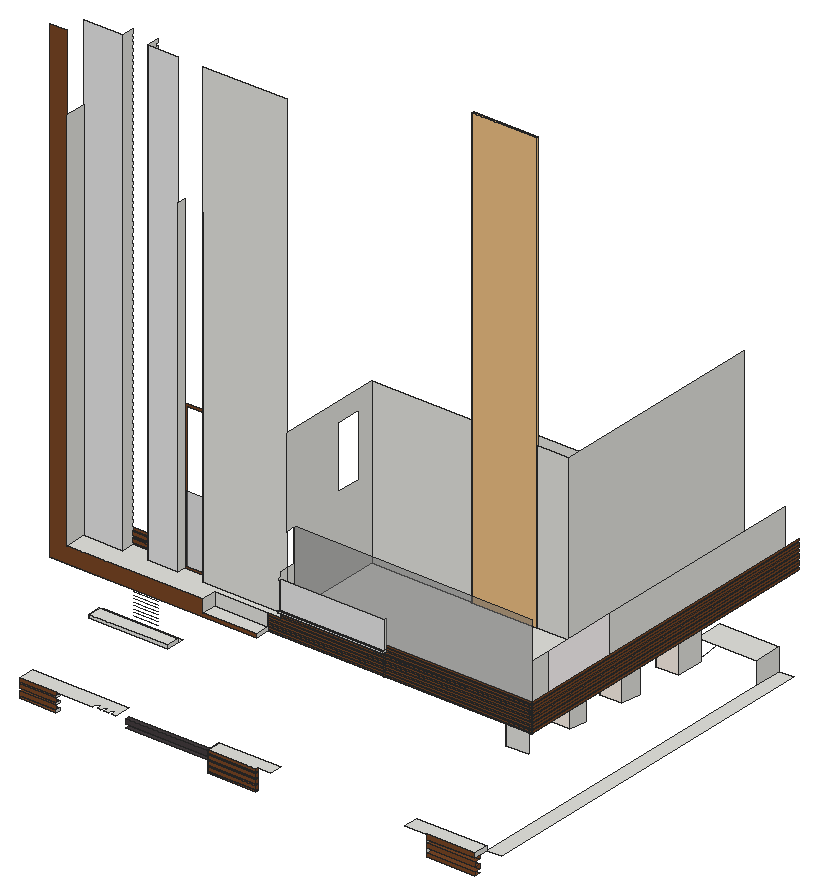
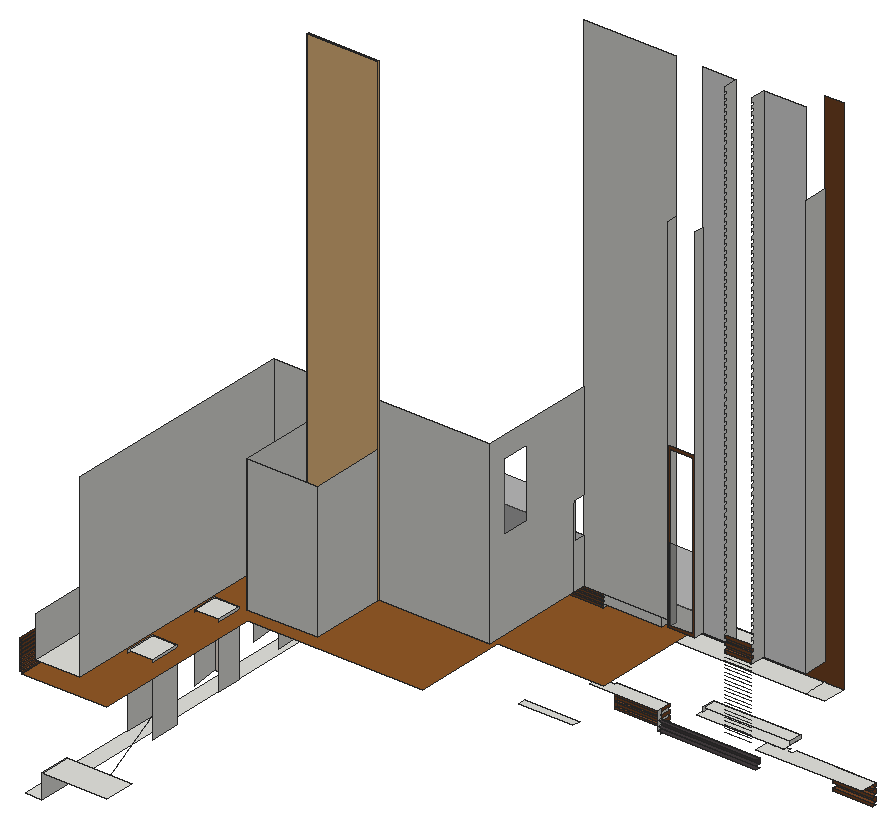
# SketchUp Ruby script. Lengths in inches.
U = 1.inch
M = Sketchup.active_model
def pt(a) = Geom::Point3d.new(a.map { |v| v * U })
def face(e, loops, mat)
  f = e.add_face(loops[0].map { |a| pt(a) })
  loops[1..].each { |l| e.add_face(l.map { |a| pt(a) }).erase! }
  f.material = f.back_material = mat if mat
  f
end
# faces: each face lists its corners as indices into pts; further lists are holes
def faces(e, pts, list, mat = nil) = list.each { |f| face(e, (f[0].is_a?(Array) ? f : [f]).map { |l| l.map { |i| pts[i] } }, mat) }
# xy, xz, yz: faces in a plane at the given z, y or x. An outline is a flat list of corners, or four numbers for a rectangle; further outlines are holes
def ring(l) = l.size == 4 ? [[l[0], l[1]], [l[2], l[1]], [l[2], l[3]], [l[0], l[3]]] : l.each_slice(2).to_a
def flat(e, list, mat, &to3) = list.each { |f| face(e, (f[0].is_a?(Array) ? f : [f]).map { |l| ring(l).map { |u, v| to3.(u, v) } }, mat) }
def xy(e, z, list, mat = nil) = flat(e, list, mat) { |x, y| [x, y, z] }
def xz(e, y, list, mat = nil) = flat(e, list, mat) { |x, z| [x, y, z] }
def yz(e, x, list, mat = nil) = flat(e, list, mat) { |y, z| [x, y, z] }
def lines(e, pts, list) = list.each { |a, b| e.add_line(pt(pts[a]), pt(pts[b])) }
# prism: a flat outline (further loops are holes) pulled along v
def prism(e, loops, v, mat = nil)
  f = face(e, loops, mat); d = Geom::Vector3d.new(v.map { |x| x * U })
  f.pushpull(f.normal.samedirection?(d) ? d.length : -d.length)
end
def box(e, o, s, mat = nil) = prism(e, [[o, [o[0] + s[0], o[1], o[2]], [o[0] + s[0], o[1] + s[1], o[2]], [o[0], o[1] + s[1], o[2]]]], [0, 0, s[2]], mat)
def at(x, y, z, deg = 0) = Geom::Transformation.translation(pt([x, y, z])) * Geom::Transformation.rotation(ORIGIN, Z_AXIS, deg.degrees)
def axes(o, x, y, z) = Geom::Transformation.new([*x, 0, *y, 0, *z, 0, *pt(o).to_a, 1])
def part(name) = M.definitions.add(name)
# library, detail: a bought-in or finely detailed component or shape, given as its bounding box
def library(name, o, s) = part(name).tap { |d| box(d.entities, o, s) }
def detail(e, o, s) = box(e.add_group.entities, o, s)
def put(e, d, t, mat = nil) = e.add_instance(d, t).tap { |i| i.material = mat if mat }
def group(e, t, mat = nil) = e.add_group.tap { |g| g.transformation = t; g.material = mat if mat }.entities
root = M.entities
M.materials.add("[0009_Linen]").color = [250, 240, 230]
M.materials.add("[0010_Snow]").color = [255, 250, 250]
M.materials.add("[Asphalt New]").color = [67, 60, 62]
M.materials.add("[Polished Concrete Old]").color = [229, 229, 229]
M.materials.add("[Translucent Glass Gray]").color = [128, 128, 128]
M.materials["[Translucent Glass Gray]"].alpha = 0.5
M.materials.add("[Wood Floor Parquet]").color = [145, 89, 39]
M.materials.add("[Wood Veneer 01]").color = [120, 70, 37]
c1 = library("Stacked entry doors",[0,-1.38,0],[114.46,3.16,780.57])
xy(root,87.39,[[455.17,254.69,541.39,258.13]],"[Wood Veneer 01]")
xy(root,87.68,[[842.13,258.13,927.67,268.51]],"[Wood Veneer 01]")
xy(root,90.67,[[455.17,254.69,541.39,258.13]],"[Wood Veneer 01]")
xy(root,91.81,[[124.44,250.88,189.05,258.13]],"[Wood Veneer 01]")
xy(root,93.96,[[842.13,258.13,927.67,268.51]],"[Wood Veneer 01]")
xy(root,94.84,[[295.6,273.26,455.17,279.68]],"[Asphalt New]")
xy(root,96.21,[[124.44,250.88,189.05,258.13]],"[Wood Veneer 01]")
xy(root,97.01,[[455.17,254.69,541.39,258.13]],"[Wood Veneer 01]")
xy(root,99.55,[[455.17,254.69,541.39,258.13]],"[Wood Veneer 01]")
xy(root,100.52,[[295.6,273.26,455.17,279.68]],"[Asphalt New]")
xy(root,101.99,[[842.13,258.13,927.67,268.51]],"[Wood Veneer 01]")
xy(root,103.18,[[124.44,250.88,189.05,258.13]],"[Wood Veneer 01]")
xy(root,105.89,[[455.17,254.69,541.39,258.13]],"[Wood Veneer 01]")
xy(root,107.59,[[124.44,250.88,189.05,258.13]],"[Wood Veneer 01]")
xy(root,108.92,[[455.17,254.69,541.39,258.13]],"[Wood Veneer 01]")
xy(root,109.42,[[295.6,273.26,455.17,279.68]],"[Asphalt New]")
xy(root,109.73,[[842.13,258.13,927.67,268.51]],"[Wood Veneer 01]")
xy(root,114.56,[[124.44,250.88,189.05,258.13]],"[Wood Veneer 01]")
xy(root,115.26,[[455.17,254.69,541.39,258.13]],"[Wood Veneer 01]")
xy(root,116.625,[[927.67,284.25,954.26,934.03]])
xy(root,117.42,[[124.44,250.88,189.05,258.13]],"[Wood Veneer 01]")
xy(root,118.74,[[455.17,254.69,541.39,258.13]],"[Wood Veneer 01]")
xy(root,124,[[124.44,250.88,253.79,250.88,253.79,258.13,262.32,258.13,262.32,250.88,268.72,250.88,268.72,258.13,274.39,258.13,274.39,250.88,281.75,250.88,281.75,258.13,287.33,258.13,287.33,250.88,295.6,250.88,295.6,279.68,124.44,279.68],[455.17,254.69,541.39,254.69,541.39,258.13,565.2,258.13,565.2,279.68,455.17,279.68],[803.4375,258.13,927.67,284.25]])
xy(root,155.125,[[821.9,884.53,927.67,934.03]])
xy(root,203.35,[[181.21,332.61,321.33,367.17]])
xy(root,209.22,[[181.21,332.61,321.33,354.61]])
xy(root,222.18,[[406.18,498.96,495.01,511.34]])
xy(root,284.1875,[[850.45,424,889.83,460.43]])
xy(root,284.375,[[850.45,516.77,889.83,551.84]])
xy(root,287.75,[[124.44,316.98,154.8,354.61],[154.8,316.98,366.22,354.61]])
xy(root,287.75,[[366.22,316.98,492.15,316.98,492.15,342.73,960.69,342.73,960.69,934.03,821.9,934.03,821.9,649.35,538.78,649.35,538.78,498.96,366.22,498.96]],"[Wood Floor Parquet]")
xy(root,290.83,[[850.45,631.85,889.83,672.61],[850.45,757.51,889.83,807.18]])
xy(root,290.83,[[492.15,342.29,701.8,342.73],[701.8,342.29,960.69,342.73],[960.69,342.73,962.51,934.03]],"[Wood Veneer 01]")
xy(root,293.61,[[397.15,316.98,492.15,342.73]])
xy(root,294,[[701.8,342.29,960.69,342.73],[960.69,342.73,962.51,934.03]],"[Wood Veneer 01]")
xy(root,296.52,[[492.15,342.29,701.8,342.73],[701.8,342.29,960.69,342.73],[960.69,342.73,962.51,934.03]],"[Wood Veneer 01]")
xy(root,299.69,[[492.15,342.29,701.8,342.73],[701.8,342.29,960.69,342.73],[960.69,342.73,962.51,934.03]],"[Wood Veneer 01]")
xy(root,302.21,[[492.15,342.29,701.8,342.73],[701.8,342.29,960.69,342.73],[960.69,342.73,962.51,934.03]],"[Wood Veneer 01]")
xy(root,305.38,[[492.15,342.29,701.8,342.73],[701.8,342.29,960.69,342.73],[960.69,342.73,962.51,934.03]],"[Wood Veneer 01]")
xy(root,307.89,[[492.15,342.29,701.8,342.73],[701.8,342.29,960.69,342.73],[960.69,342.73,962.51,934.03]],"[Wood Veneer 01]")
xy(root,311.07,[[492.15,342.29,701.8,342.73],[701.8,342.29,960.69,342.73],[960.69,342.73,962.51,934.03]],"[Wood Veneer 01]")
xy(root,313.58,[[492.15,342.29,701.8,342.73],[701.8,342.29,960.69,342.73],[960.69,342.73,962.51,934.03]],"[Wood Veneer 01]")
xy(root,316.375,[[154.8,316.98,397.15,316.98,397.15,342.73,492.15,342.73,492.15,342.29,515.24,342.29,515.24,354.61,366.22,354.61,366.22,370.17,322.47,370.17,322.47,354.61,268.36,354.61,268.36,378.04,224.18,378.04,224.18,354.61,154.8,354.61],[515.24,373.53,937.99,373.53,937.99,543.54,810.09,543.54,810.09,667.11,695.625,667.11,695.625,543.54,515.24,543.54],[865.61,543.54,937.99,934.03]])
xy(root,316.75,[[701.8,342.29,960.69,342.73],[960.69,342.73,962.51,934.03]],"[Wood Veneer 01]")
xy(root,319.27,[[515.24,342.29,701.8,342.73],[701.8,342.29,960.69,342.73],[960.69,342.73,962.51,934.03]],"[Wood Veneer 01]")
xy(root,321.94,[[224.18,374.04,268.36,378.04]],"[Wood Veneer 01]")
xy(root,322.44,[[515.24,342.29,701.8,342.73],[701.8,342.29,960.69,342.73],[960.69,342.73,962.51,934.03]],"[Wood Veneer 01]")
xy(root,324.96,[[515.24,342.29,701.8,342.73],[701.8,342.29,960.69,342.73],[960.69,342.73,962.51,934.03]],"[Wood Veneer 01]")
xy(root,327.89,[[515.24,336.36,701.8,342.29]])
xy(root,327.96,[[224.18,374.04,268.36,378.04]],"[Wood Veneer 01]")
xy(root,328.13,[[701.8,342.29,960.69,342.73],[960.69,342.73,962.51,934.03]],"[Wood Veneer 01]")
xy(root,330.375,[[515.24,336.36,701.8,339.61]])
xy(root,330.64,[[701.8,342.29,960.69,342.73],[960.69,342.73,962.51,934.03]],"[Wood Veneer 01]")
xy(root,332.82,[[224.18,374.04,268.36,378.04]],"[Wood Veneer 01]")
xy(root,333.82,[[701.8,342.29,960.69,342.73],[960.69,342.73,962.51,934.03]],"[Wood Veneer 01]")
xy(root,336.33,[[701.8,342.29,960.69,342.73],[960.69,342.73,962.51,934.03]],"[Wood Veneer 01]")
xy(root,338.84,[[224.18,374.04,268.36,378.04]],"[Wood Veneer 01]")
xz(root,250.88,[[124.44,96.21,189.05,103.18],[124.44,107.59,189.05,114.56],[124.44,117.42,189.05,124]],"[Wood Veneer 01]")
xz(root,254.69,[[455.17,90.67,541.39,97.01],[455.17,99.55,541.39,105.89],[455.17,108.92,541.39,115.26],[455.17,118.74,541.39,124]],"[Wood Veneer 01]")
xz(root,258.13,[[455.17,87.39,541.39,90.67],[842.13,87.68,927.67,93.96],[124.44,91.81,189.05,96.21],[455.17,97.01,541.39,99.55],[842.13,101.99,927.67,109.73],
  [124.44,103.18,189.05,107.59],[455.17,105.89,541.39,108.92],[124.44,114.56,189.05,117.42],[455.17,115.26,541.39,118.74],[842.13,115.72,927.67,116.625,927.67,124,842.13,124]],"[Wood Veneer 01]")
xz(root,268.51,[[842.13,93.96,927.67,101.99],[842.13,109.73,927.67,109.73,927.67,116.625,842.13,115.72]],"[Wood Veneer 01]")
xz(root,273.26,[[295.6,100.52,455.17,109.42]],"[Asphalt New]")
xz(root,316.98,[[124.44,287.75,492.15,287.75,492.15,293.61,397.15,293.61,397.15,316.375,154.8,316.375,154.8,1137.19,124.44,1137.19]],"[Wood Veneer 01]")
xz(root,332.61,[[181.21,203.35,321.33,209.22]])
xz(root,336.36,[[515.24,327.89,701.8,330.375]],"[Polished Concrete Old]")
xz(root,339.61,[[515.24,330.375,701.8,380.42]],"[Polished Concrete Old]")
xz(root,342.29,[[492.15,290.83,701.8,290.83,701.8,294,492.15,293.61],[701.8,290.83,960.69,294],[492.15,296.52,701.8,299.69],[701.8,296.52,960.69,299.69],[492.15,302.21,701.8,305.38],
  [701.8,302.21,960.69,305.38],[492.15,307.89,701.8,311.07],[701.8,307.89,960.69,311.07],[492.15,313.58,701.8,313.58,701.8,316.75,515.24,316.375,492.15,316.375],[701.8,313.58,960.69,316.75],
  [515.24,319.27,701.8,322.44],[701.8,319.27,960.69,322.44],[515.24,324.96,701.8,327.89],[701.8,324.96,960.69,328.13],[701.8,330.64,960.69,333.82],
  [701.8,336.33,960.69,339.5]],"[Wood Veneer 01]")
xz(root,342.73,[[397.15,293.61,492.15,316.375]])
xz(root,342.73,[[492.15,287.75,701.8,288.32],[701.8,287.75,960.69,288.32],[492.15,288.32,701.8,290.83],[701.8,288.32,960.69,290.83],[960.69,290.83,962.51,294],
  [492.15,293.61,701.8,294,701.8,296.52,492.15,296.52],[701.8,294,960.69,296.52],[960.69,296.52,962.51,299.69],[492.15,299.69,701.8,302.21],[701.8,299.69,960.69,302.21],
  [960.69,302.21,962.51,305.38],[492.15,305.38,701.8,307.89],[701.8,305.38,960.69,307.89],[960.69,307.89,962.51,311.07],[492.15,311.07,701.8,313.58],
  [701.8,311.07,960.69,313.58],[960.69,313.58,962.51,316.75],[515.24,316.375,701.8,316.75,701.8,319.27,515.24,319.27],[701.8,316.75,960.69,319.27],[960.69,319.27,962.51,322.44],
  [515.24,322.44,701.8,324.96],[701.8,322.44,960.69,324.96],[960.69,324.96,962.51,328.13],[701.8,328.13,960.69,330.64],[960.69,330.64,962.51,333.82],
  [701.8,333.82,960.69,336.33],[960.69,336.33,962.51,339.5]],"[Wood Veneer 01]")
xz(root,354.61,[[366.22,316.375,515.24,1137.19]])
xz(root,354.61,[[154.8,316.375,224.18,1137.19],[268.36,316.375,322.47,1137.19]],"[Polished Concrete Old]")
xz(root,370.17,[[326.19,320.1,362.49,440.01]],"[Translucent Glass Gray]")
xz(root,370.17,[[[322.47,316.375,366.22,579.93],[326.19,320.1,362.49,576.21]]],"[Wood Veneer 01]")
xz(root,373.53,[[515.24,316.375,937.99,449.0625]],"[Translucent Glass Gray]")
xz(root,374.04,[[224.18,321.94,268.36,327.96],[224.18,332.82,268.36,338.84]],"[Wood Veneer 01]")
xz(root,378.04,[[224.18,316.375,268.36,317.09],[224.18,317.09,268.36,321.94],[224.18,327.96,268.36,332.82],[224.18,338.84,268.36,343.69]],"[Wood Veneer 01]")
xz(root,424,[[850.45,195.12,889.83,284.1875]])
xz(root,516.77,[[850.45,195.12,889.83,284.375]],"[0009_Linen]")
xz(root,543.54,[[515.24,316.375,695.625,316.375,695.625,534.49,810.09,534.49,810.09,316.375,865.61,316.375,865.61,605.77,515.24,605.77]])
xz(root,631.85,[[850.45,185.07,889.83,290.83]],"[0009_Linen]")
xz(root,667.11,[[695.625,316.375,810.09,534.49]])
xz(root,757.51,[[850.45,174.63,889.83,290.83]],"[0009_Linen]")
yz(root,154.8,[[316.98,316.375,354.61,1001.72]])
yz(root,181.21,[[332.61,203.35,354.61,209.22]])
yz(root,189.05,[[250.88,91.81,258.13,96.21],[250.88,103.18,258.13,107.59],[250.88,114.56,258.13,117.42]])
yz(root,224.18,[[354.61,316.375,378.04,316.375,378.04,321.94,374.04,321.94,374.04,327.96,378.04,327.96,378.04,332.82,374.04,332.82,374.04,338.84,378.04,338.84,378.04,343.69,374.04,343.69,374.04,349.71,378.04,349.71,378.04,354.57,374.04,354.57,374.04,360.59,378.04,360.59,378.04,365.44,374.04,365.44,374.04,371.46,378.04,371.46,378.04,376.32,374.04,376.32,374.04,382.34,378.04,382.34,378.04,387.19,374.04,387.19,374.04,393.21,378.04,393.21,378.04,398.07,374.04,398.07,374.04,404.09,378.04,404.09,378.04,408.94,374.04,408.94,374.04,414.96,378.04,414.96,378.04,419.82,374.04,419.82,374.04,425.84,378.04,425.84,378.04,430.69,374.04,430.69,374.04,436.71,378.04,436.71,378.04,441.57,374.04,441.57,374.04,447.59,378.04,447.59,378.04,452.44,374.04,452.44,374.04,458.46,378.04,458.46,378.04,463.32,374.04,463.32,374.04,469.34,378.04,469.34,378.04,474.19,374.04,474.19,374.04,480.21,378.04,480.21,378.04,485.07,374.04,485.07,374.04,491.09,378.04,491.09,378.04,495.94,374.04,495.94,374.04,501.96,378.04,501.96,378.04,507.44,374.04,507.44,374.04,513.46,378.04,513.46,378.04,518.94,374.04,518.94,374.04,524.96,378.04,524.96,378.04,530.44,374.04,530.44,374.04,536.46,378.04,536.46,378.04,541.94,374.04,541.94,374.04,547.96,378.04,547.96,378.04,553.44,374.04,553.44,374.04,559.46,378.04,559.46,378.04,564.94,374.04,564.94,374.04,570.96,378.04,570.96,378.04,576.44,374.04,576.44,374.04,582.46,378.04,582.46,378.04,587.94,374.04,587.94,374.04,593.96,378.04,593.96,378.04,599.44,374.04,599.44,374.04,605.46,378.04,605.46,378.04,610.94,374.04,610.94,374.04,616.96,378.04,616.96,378.04,622.44,374.04,622.44,374.04,628.46,378.04,628.46,378.04,633.94,374.04,633.94,374.04,639.96,378.04,639.96,378.04,645.44,374.04,645.44,374.04,651.46,378.04,651.46,378.04,656.94,374.04,656.94,374.04,662.96,378.04,662.96,378.04,668.44,374.04,668.44,374.04,674.46,378.04,674.46,378.04,679.94,374.04,679.94,374.04,685.96,378.04,685.96,378.04,691.44,374.04,691.44,374.04,697.46,378.04,697.46,378.04,702.94,374.04,702.94,374.04,708.96,378.04,708.96,378.04,714.44,374.04,714.44,374.04,720.46,378.04,720.46,378.04,725.94,374.04,725.94,374.04,731.96,378.04,731.96,378.04,737.44,374.04,737.44,374.04,743.46,378.04,743.46,378.04,748.94,374.04,748.94,374.04,754.96,378.04,754.96,378.04,760.44,374.04,760.44,374.04,766.46,378.04,766.46,378.04,771.94,374.04,771.94,374.04,777.96,378.04,777.96,378.04,783.44,374.04,783.44,374.04,789.46,378.04,789.46,378.04,794.94,374.04,794.94,374.04,800.96,378.04,800.96,378.04,806.44,374.04,806.44,374.04,812.46,378.04,812.46,378.04,817.94,374.04,817.94,374.04,823.96,378.04,823.96,378.04,829.44,374.04,829.44,374.04,835.46,378.04,835.46,378.04,840.94,374.04,840.94,374.04,846.96,378.04,846.96,378.04,851.5,374.04,851.5,374.04,857.52,378.04,857.52,378.04,862.07,374.04,862.07,374.04,868.09,378.04,868.09,378.04,872.63,374.04,872.63,374.04,878.65,378.04,878.65,378.04,883.19,374.04,883.19,374.04,889.21,378.04,889.21,378.04,893.75,374.04,893.75,374.04,899.77,378.04,899.77,378.04,904.32,374.04,904.32,374.04,910.34,378.04,910.34,378.04,914.88,374.04,914.88,374.04,920.9,378.04,920.9,378.04,925.44,374.04,925.44,374.04,931.46,378.04,931.46,378.04,936,374.04,936,374.04,942.02,378.04,942.02,378.04,946.57,374.04,946.57,374.04,952.59,378.04,952.59,378.04,957.13,374.04,957.13,374.04,963.15,378.04,963.15,378.04,967.69,374.04,967.69,374.04,973.71,378.04,973.71,378.04,978.25,374.04,978.25,374.04,984.27,378.04,984.27,378.04,988.82,374.04,988.82,374.04,994.84,378.04,994.84,378.04,999.38,374.04,999.38,374.04,1005.4,378.04,1005.4,378.04,1009.94,374.04,1009.94,374.04,1015.96,378.04,1015.96,378.04,1020.5,374.04,1020.5,374.04,1026.52,378.04,1026.52,378.04,1031.07,374.04,1031.07,374.04,1037.09,378.04,1037.09,378.04,1041.63,374.04,1041.63,374.04,1047.65,378.04,1047.65,378.04,1052.19,374.04,1052.19,374.04,1058.21,378.04,1058.21,378.04,1062.75,374.04,1062.75,374.04,1068.77,378.04,1068.77,378.04,1073.32,374.04,1073.32,374.04,1079.34,378.04,1079.34,378.04,1083.88,374.04,1083.88,374.04,1089.9,378.04,1089.9,378.04,1094.44,374.04,1094.44,374.04,1100.46,378.04,1100.46,378.04,1105,374.04,1105,374.04,1111.02,378.04,1111.02,378.04,1115.76,374.04,1115.76,374.04,1120.3,378.04,1120.3,378.04,1124.95,374.04,1124.95,374.04,1129.68,378.04,1129.68,378.04,1137.19,354.61,1137.19]])
yz(root,268.36,[[354.61,316.375,354.61,1137.19,378.04,1137.19,378.04,1129.68,374.04,1129.68,374.04,1124.95,378.04,1124.95,378.04,1120.3,374.04,1120.3,374.04,1115.76,378.04,1115.76,378.04,1111.02,374.04,1111.02,374.04,1105,378.04,1105,378.04,1100.46,374.04,1100.46,374.04,1094.44,378.04,1094.44,378.04,1089.9,374.04,1089.9,374.04,1083.88,378.04,1083.88,378.04,1079.34,374.04,1079.34,374.04,1073.32,378.04,1073.32,378.04,1068.77,374.04,1068.77,374.04,1062.75,378.04,1062.75,378.04,1058.21,374.04,1058.21,374.04,1052.19,378.04,1052.19,378.04,1047.65,374.04,1047.65,374.04,1041.63,378.04,1041.63,378.04,1037.09,374.04,1037.09,374.04,1031.07,378.04,1031.07,378.04,1026.52,374.04,1026.52,374.04,1020.5,378.04,1020.5,378.04,1015.96,374.04,1015.96,374.04,1009.94,378.04,1009.94,378.04,1005.4,374.04,1005.4,374.04,999.38,378.04,999.38,378.04,994.84,374.04,994.84,374.04,988.82,378.04,988.82,378.04,984.27,374.04,984.27,374.04,978.25,378.04,978.25,378.04,973.71,374.04,973.71,374.04,967.69,378.04,967.69,378.04,963.15,374.04,963.15,374.04,957.13,378.04,957.13,378.04,952.59,374.04,952.59,374.04,946.57,378.04,946.57,378.04,942.02,374.04,942.02,374.04,936,378.04,936,378.04,931.46,374.04,931.46,374.04,925.44,378.04,925.44,378.04,920.9,374.04,920.9,374.04,914.88,378.04,914.88,378.04,910.34,374.04,910.34,374.04,904.32,378.04,904.32,378.04,899.77,374.04,899.77,374.04,893.75,378.04,893.75,378.04,889.21,374.04,889.21,374.04,883.19,378.04,883.19,378.04,878.65,374.04,878.65,374.04,872.63,378.04,872.63,378.04,868.09,374.04,868.09,374.04,862.07,378.04,862.07,378.04,857.52,374.04,857.52,374.04,851.5,378.04,851.5,378.04,846.96,374.04,846.96,374.04,840.94,378.04,840.94,378.04,835.46,374.04,835.46,374.04,829.44,378.04,829.44,378.04,823.96,374.04,823.96,374.04,817.94,378.04,817.94,378.04,812.46,374.04,812.46,374.04,806.44,378.04,806.44,378.04,800.96,374.04,800.96,374.04,794.94,378.04,794.94,378.04,789.46,374.04,789.46,374.04,783.44,378.04,783.44,378.04,777.96,374.04,777.96,374.04,771.94,378.04,771.94,378.04,766.46,374.04,766.46,374.04,760.44,378.04,760.44,378.04,754.96,374.04,754.96,374.04,748.94,378.04,748.94,378.04,743.46,374.04,743.46,374.04,737.44,378.04,737.44,378.04,731.96,374.04,731.96,374.04,725.94,378.04,725.94,378.04,720.46,374.04,720.46,374.04,714.44,378.04,714.44,378.04,708.96,374.04,708.96,374.04,702.94,378.04,702.94,378.04,697.46,374.04,697.46,374.04,691.44,378.04,691.44,378.04,685.96,374.04,685.96,374.04,679.94,378.04,679.94,378.04,674.46,374.04,674.46,374.04,668.44,378.04,668.44,378.04,662.96,374.04,662.96,374.04,656.94,378.04,656.94,378.04,651.46,374.04,651.46,374.04,645.44,378.04,645.44,378.04,639.96,374.04,639.96,374.04,633.94,378.04,633.94,378.04,628.46,374.04,628.46,374.04,622.44,378.04,622.44,378.04,616.96,374.04,616.96,374.04,610.94,378.04,610.94,378.04,605.46,374.04,605.46,374.04,599.44,378.04,599.44,378.04,593.96,374.04,593.96,374.04,587.94,378.04,587.94,378.04,582.46,374.04,582.46,374.04,576.44,378.04,576.44,378.04,570.96,374.04,570.96,374.04,564.94,378.04,564.94,378.04,559.46,374.04,559.46,374.04,553.44,378.04,553.44,378.04,547.96,374.04,547.96,374.04,541.94,378.04,541.94,378.04,536.46,374.04,536.46,374.04,530.44,378.04,530.44,378.04,524.96,374.04,524.96,374.04,518.94,378.04,518.94,378.04,513.46,374.04,513.46,374.04,507.44,378.04,507.44,378.04,501.96,374.04,501.96,374.04,495.94,378.04,495.94,378.04,491.09,374.04,491.09,374.04,485.07,378.04,485.07,378.04,480.21,374.04,480.21,374.04,474.19,378.04,474.19,378.04,469.34,374.04,469.34,374.04,463.32,378.04,463.32,378.04,458.46,374.04,458.46,374.04,452.44,378.04,452.44,378.04,447.59,374.04,447.59,374.04,441.57,378.04,441.57,378.04,436.71,374.04,436.71,374.04,430.69,378.04,430.69,378.04,425.84,374.04,425.84,374.04,419.82,378.04,419.82,378.04,414.96,374.04,414.96,374.04,408.94,378.04,408.94,378.04,404.09,374.04,404.09,374.04,398.07,378.04,398.07,378.04,393.21,374.04,393.21,374.04,387.19,378.04,387.19,378.04,382.34,374.04,382.34,374.04,376.32,378.04,376.32,378.04,371.46,374.04,371.46,374.04,365.44,378.04,365.44,378.04,360.59,374.04,360.59,374.04,354.57,378.04,354.57,378.04,349.71,374.04,349.71,374.04,343.69,378.04,343.69,378.04,338.84,374.04,338.84,374.04,332.82,378.04,332.82,378.04,327.96,374.04,327.96,374.04,321.94,378.04,321.94,378.04,316.375]])
yz(root,321.33,[[332.61,203.35,354.61,209.22]])
yz(root,322.47,[[354.61,316.375,370.17,904.26]])
yz(root,366.22,[[354.61,316.375,370.17,904.26]])
yz(root,397.15,[[316.98,293.61,342.73,316.375]])
yz(root,455.17,[[258.13,87.39,273.26,90.67],[273.26,94.84,279.68,100.52],[258.13,97.01,273.26,99.55],[273.26,100.52,279.68,109.42],[258.13,105.89,273.26,108.92],
  [273.26,109.42,279.68,124],[258.13,115.26,273.26,118.74]])
yz(root,455.17,[[254.69,90.67,273.26,97.01],[254.69,99.55,273.26,105.89],[254.69,108.92,273.26,115.26],[254.69,118.74,273.26,124]],"[Wood Veneer 01]")
yz(root,492.15,[[316.98,287.75,342.73,287.75,342.73,290.83,342.29,290.83,342.29,293.61,316.98,293.61]])
yz(root,492.15,[[342.29,296.52,342.73,299.69],[342.29,302.21,342.73,305.38],[342.29,307.89,342.73,311.07],[342.29,313.58,342.73,316.375]],"[Wood Veneer 01]")
yz(root,515.24,[[342.73,316.375,342.73,319.27,342.29,319.27,342.29,322.44,342.73,322.44,342.73,324.96,342.29,324.96,342.29,327.89,336.36,327.89,336.36,330.375,339.61,330.375,339.61,380.42,336.73,380.42,336.73,381.83,342.29,381.83,342.29,385,342.73,385,342.73,386.71,342.29,386.71,342.29,390.25,354.61,390.25,354.61,316.375],[354.61,316.375,354.61,390.25,371.82,390.25,371.82,449.0625,373.53,449.0625,373.53,316.375],[[373.53,316.375,543.54,316.375,543.54,605.77,354.61,605.77,354.61,449.0625,373.53,449.0625],[469.55,461.11,514.92,571.62]]])
yz(root,541.39,[[254.69,90.67,258.13,97.01],[254.69,99.55,258.13,105.89],[254.69,108.92,258.13,115.26],[254.69,118.74,258.13,124]],"[Wood Veneer 01]")
yz(root,695.625,[[543.54,316.375,667.11,534.49]])
yz(root,701.8,[[336.36,327.89,342.29,327.89,342.29,328.13,342.73,328.13,342.73,330.375,336.36,330.375],[339.61,330.375,342.73,330.375,342.73,330.64,342.29,330.64,342.29,333.82,342.73,333.82,342.73,336.33,342.29,336.33,342.29,339.5,342.73,339.5,342.73,342.02,342.29,342.02,342.29,345.19,342.73,345.19,342.73,347.71,342.29,347.71,342.29,350.88,342.73,350.88,342.73,353.39,342.29,353.39,342.29,356.57,342.73,356.57,342.73,359.08,342.29,359.08,342.29,362.25,342.73,362.25,342.73,364.77,342.29,364.77,342.29,367.94,342.73,367.94,342.73,370.46,342.29,370.46,342.29,373.63,342.73,373.63,342.73,376.14,342.29,376.14,342.29,379.32,342.73,379.32,342.73,380.42,339.61,380.42]])
yz(root,810.09,[[543.54,316.375,667.11,534.49]])
yz(root,842.13,[[258.13,93.96,268.51,101.99],[258.13,109.73,268.51,115.72]])
yz(root,850.45,[[757.51,174.63,807.18,290.83],[631.85,185.07,672.61,290.83],[424,195.12,460.43,284.1875],[516.77,195.12,551.84,284.375]])
yz(root,865.61,[[543.54,316.375,934.03,605.77]])
yz(root,889.83,[[757.51,174.63,807.18,290.83],[672.61,180.31,672.61,290.83,631.85,290.83,631.85,185.07],[551.84,191.02,551.84,284.375,516.77,284.375,516.77,195.12]])
yz(root,927.67,[[258.13,116.625,284.25,124],[884.53,116.625,934.03,155.125]])
yz(root,937.99,[[373.53,316.375,408.2,382.72],[543.54,316.375,934.03,382.72]])
yz(root,937.99,[[408.2,316.375,543.54,382.72]],"[0010_Snow]")
yz(root,960.69,[[342.73,287.75,934.03,288.32],[342.29,290.83,342.73,294],[342.29,296.52,342.73,299.69],[342.29,302.21,342.73,305.38],[342.29,307.89,342.73,311.07],
  [342.29,313.58,342.73,316.75],[342.29,319.27,342.73,322.44],[342.29,324.96,342.73,328.13],[342.29,330.64,342.73,333.82],[342.29,336.33,342.73,339.5]])
yz(root,960.69,[[342.73,288.32,934.03,290.83],[342.73,294,934.03,296.52],[342.73,299.69,934.03,302.21],[342.73,305.38,934.03,307.89],[342.73,311.07,934.03,313.58],
  [342.73,316.75,934.03,319.27],[342.73,322.44,934.03,324.96],[342.73,328.13,934.03,330.64],[342.73,333.82,934.03,336.33]],"[Wood Veneer 01]")
yz(root,962.51,[[342.73,290.83,934.03,294],[342.73,296.52,934.03,299.69],[342.73,302.21,934.03,305.38],[342.73,307.89,934.03,311.07],[342.73,313.58,934.03,316.75],
  [342.73,319.27,934.03,322.44],[342.73,324.96,934.03,328.13],[342.73,330.64,934.03,333.82],[342.73,336.33,934.03,339.5]],"[Wood Veneer 01]")
p = [[842.13,268.51,115.72],[927.67,268.51,116.625],[927.67,258.13,116.625],[842.13,258.13,115.72],[701.8,342.73,294],[492.15,342.73,293.61],
  [492.15,342.29,293.61],[701.8,342.29,294],[701.8,342.73,316.75],[515.24,342.73,316.375],[515.24,342.29,316.375],[701.8,342.29,316.75],
  [224.18,378.04,311.07],[268.36,378.04,311.07],[224.18,378.04,300.19],[268.36,378.04,300.19],[268.36,378.04,306.21],[224.18,378.04,306.21],
  [224.18,378.04,289.32],[268.36,378.04,289.32],[268.36,378.04,295.34],[224.18,378.04,295.34],[224.18,378.04,278.44],[268.36,378.04,278.44],
  [268.36,378.04,284.46],[224.18,378.04,284.46],[224.18,378.04,267.57],[268.36,378.04,267.57],[268.36,378.04,273.59],[224.18,378.04,273.59],
  [224.18,378.04,256.69],[268.36,378.04,256.69],[268.36,378.04,262.71],[224.18,378.04,262.71],[224.18,378.04,245.82],[268.36,378.04,245.82],
  [268.36,378.04,251.84],[224.18,378.04,251.84],[224.18,378.04,234.94],[268.36,378.04,234.94],[268.36,378.04,240.96],[224.18,378.04,240.96],
  [224.18,378.04,224.07],[268.36,378.04,224.07],[268.36,378.04,230.09],[224.18,378.04,230.09],[224.18,378.04,213.19],[268.36,378.04,213.19],
  [268.36,378.04,219.21],[224.18,378.04,219.21],[224.18,378.04,202.32],[268.36,378.04,202.32],[268.36,378.04,208.34],[224.18,378.04,208.34],
  [889.83,757.51,174.63],[856.64,884.53,155.125]]
faces(root,p,[[0,1,2,3],[4,5,6,7],[8,9,10,11]],"[Wood Veneer 01]")
lines(root,p,[[12,13],[14,15],[16,17],[18,19],[20,21],[22,23],[24,25],[26,27],[28,29],[30,31],[32,33],[34,35],
  [36,37],[38,39],[40,41],[42,43],[44,45],[46,47],[48,49],[50,51],[52,53],[54,55]])
put(root,c1,at(695.625,543.54,316.375))
